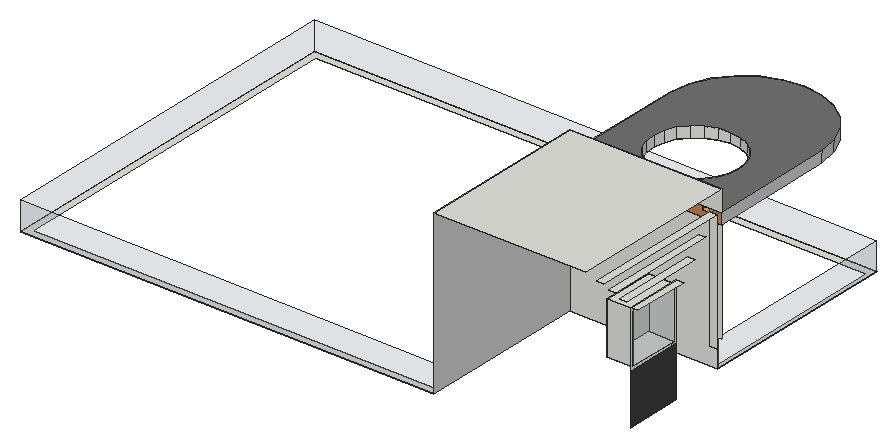
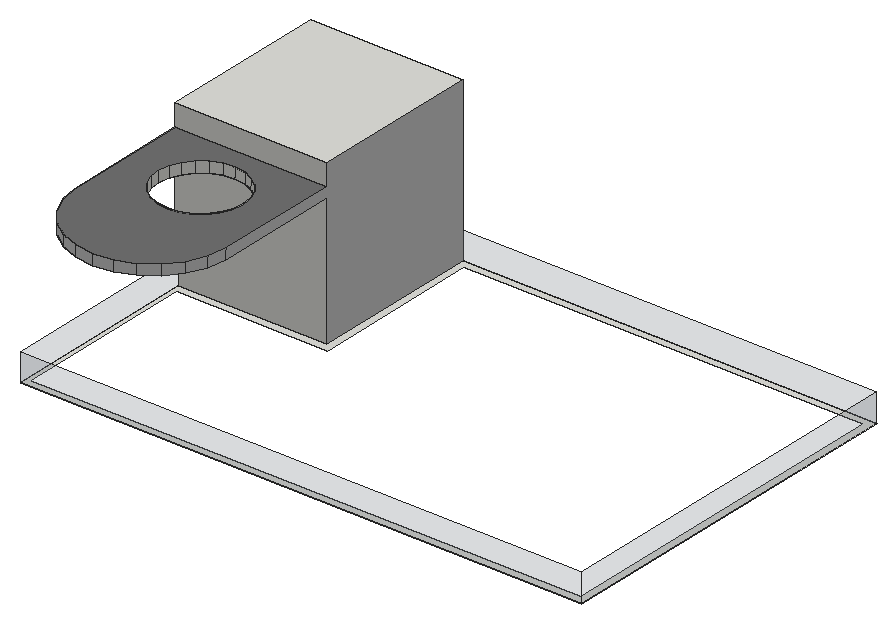
# SketchUp Ruby script. Lengths in inches.
U = 1.inch
M = Sketchup.active_model
def pt(a) = Geom::Point3d.new(a.map { |v| v * U })
def face(e, loops, mat)
  f = e.add_face(loops[0].map { |a| pt(a) })
  loops[1..].each { |l| e.add_face(l.map { |a| pt(a) }).erase! }
  f.material = f.back_material = mat if mat
  f
end
# faces: each face lists its corners as indices into pts; further lists are holes
def faces(e, pts, list, mat = nil) = list.each { |f| face(e, (f[0].is_a?(Array) ? f : [f]).map { |l| l.map { |i| pts[i] } }, mat) }
# xy, xz, yz: faces in a plane at the given z, y or x. An outline is a flat list of corners, or four numbers for a rectangle; further outlines are holes
def ring(l) = l.size == 4 ? [[l[0], l[1]], [l[2], l[1]], [l[2], l[3]], [l[0], l[3]]] : l.each_slice(2).to_a
def flat(e, list, mat, &to3) = list.each { |f| face(e, (f[0].is_a?(Array) ? f : [f]).map { |l| ring(l).map { |u, v| to3.(u, v) } }, mat) }
def xy(e, z, list, mat = nil) = flat(e, list, mat) { |x, y| [x, y, z] }
def xz(e, y, list, mat = nil) = flat(e, list, mat) { |x, z| [x, y, z] }
def yz(e, x, list, mat = nil) = flat(e, list, mat) { |y, z| [x, y, z] }
def lines(e, pts, list) = list.each { |a, b| e.add_line(pt(pts[a]), pt(pts[b])) }
# prism: a flat outline (further loops are holes) pulled along v
def prism(e, loops, v, mat = nil)
  f = face(e, loops, mat); d = Geom::Vector3d.new(v.map { |x| x * U })
  f.pushpull(f.normal.samedirection?(d) ? d.length : -d.length)
end
def box(e, o, s, mat = nil) = prism(e, [[o, [o[0] + s[0], o[1], o[2]], [o[0] + s[0], o[1] + s[1], o[2]], [o[0], o[1] + s[1], o[2]]]], [0, 0, s[2]], mat)
def at(x, y, z, deg = 0) = Geom::Transformation.translation(pt([x, y, z])) * Geom::Transformation.rotation(ORIGIN, Z_AXIS, deg.degrees)
def axes(o, x, y, z) = Geom::Transformation.new([*x, 0, *y, 0, *z, 0, *pt(o).to_a, 1])
def part(name) = M.definitions.add(name)
# library, detail: a bought-in or finely detailed component or shape, given as its bounding box
def library(name, o, s) = part(name).tap { |d| box(d.entities, o, s) }
def detail(e, o, s) = box(e.add_group.entities, o, s)
def put(e, d, t, mat = nil) = e.add_instance(d, t).tap { |i| i.material = mat if mat }
def group(e, t, mat = nil) = e.add_group.tap { |g| g.transformation = t; g.material = mat if mat }.entities
root = M.entities
M.materials.add("Glass_Basic_01").color = [161, 173, 186]
M.materials["Glass_Basic_01"].alpha = 0.25
M.materials.add("M05_Graphite_Haze").color = [114, 114, 114]
M.materials.add("ThomThom - Hat3").color = [58, 58, 58]
M.materials.add("Wood_Veneer_15_1K").color = [173, 116, 75]
M.materials.add("[_0128_White_]").color = [200, 200, 200]
c1 = library("Sphere Light\#1",[-3.43,-3.43,-3.43],[6.86,6.86,6.86])
c2 = library("Sphere Light",[-3.0625,-3.0625,-3.0625],[6.125,6.125,6.125])
c3 = library("Sphere Light\#2",[-2.85,-2.85,-2.85],[5.7,5.7,5.7])
xy(root,270,[[[0,0,351.33,0,351.33,144,477,144,477,312,0,312],[6,6,6,306,474,306,474,150,345.33,150,345.33,6]]])
xy(root,314,[[458.06,50,480,94]])
xy(root,358,[[458.06,50,480,94]])
xy(root,360,[[480,48,486,96]])
xy(root,372,[[480,36,486,108]])
xy(root,381,[[367.15,152.16,367.91,152.34,368.6,152.71,369.17,153.25,369.58,153.92,369.8,154.67,369.82,155.45,369.64,156.21,369.26,156.9,368.73,157.47,368.06,157.88,367.31,158.1,366.52,158.125,365.76,157.94,365.07,157.57,364.51,157.03,364.1,156.36,363.875,155.61,363.85,154.83,364.03,154.07,364.41,153.38,364.95,152.81,365.61,152.4,366.37,152.18],[460.92,152.16,461.68,152.34,462.37,152.71,462.9375,153.25,463.35,153.92,463.57,154.67,463.59,155.45,463.41,156.21,463.03,156.9,462.49,157.47,461.83,157.88,461.08,158.1,460.29,158.125,459.53,157.94,458.84,157.57,458.28,157.03,457.87,156.36,457.64,155.61,457.62,154.83,457.8,154.07,458.18,153.38,458.72,152.81,459.38,152.4,460.13,152.18],[415.67,261.6,416.44,261.71,417.17,262.01,417.79,262.48,418.26,263.1,418.56,263.83,418.67,264.6,418.56,265.38,418.26,266.1,417.79,266.73,417.17,267.2,416.44,267.5,415.67,267.6,414.89,267.5,414.17,267.2,413.55,266.73,413.07,266.1,412.77,265.38,412.67,264.6,412.77,263.83,413.07,263.1,413.55,262.48,414.17,262.01,414.89,261.71]])
xy(root,381,[[[351.33,144,351.33,250.65,354.16,266.71,360.9375,281.55,371.22,294.2,384.35,303.875,399.49,309.94,415.67,312,431.84,309.94,446.98,303.875,460.11,294.2,470.4,281.55,477.17,266.71,480,250.65,480,144],[415.67,161.33,424.98,162.55,433.67,166.15,441.12,171.87,446.84,179.33,450.44,188.01,451.67,197.33,450.44,206.64,446.84,215.33,441.12,222.78,433.67,228.5,424.98,232.1,415.67,233.33,406.35,232.1,397.67,228.5,390.21,222.78,384.49,215.33,380.89,206.64,379.67,197.33,380.89,188.01,384.49,179.33,390.21,171.87,397.67,166.15,406.35,162.55],[409.67,279.92,421.67,291.92]]],"Wood_Veneer_15_1K")
xy(root,384,[[480,24,486,120]])
xy(root,390,[[[351.33,144,480,144,480,250.65,477.17,266.71,470.4,281.55,460.11,294.2,446.98,303.875,431.84,309.94,415.67,312,399.49,309.94,384.35,303.875,371.22,294.2,360.9375,281.55,354.16,266.71,351.33,250.65],[415.67,161.33,406.35,162.55,397.67,166.15,390.21,171.87,384.49,179.33,380.89,188.01,379.67,197.33,380.89,206.64,384.49,215.33,390.21,222.78,397.67,228.5,406.35,232.1,415.67,233.33,424.98,232.1,433.67,228.5,441.12,222.78,446.84,215.33,450.44,206.64,451.67,197.33,450.44,188.01,446.84,179.33,441.12,171.87,433.67,166.15,424.98,162.55]]],"M05_Graphite_Haze")
xy(root,396,[[480,12,486,132]])
xy(root,408,[[351.33,0,480,144]])
xz(root,0,[[0,270,351.33,294]],"Glass_Basic_01")
xz(root,50,[[458.06,314,480,358]])
xz(root,94,[[458.06,314,480,358]])
xz(root,132,[[480,294,486,396]])
xz(root,144,[[351.33,270,351.33,381,480,381,480,294,477,294,477,270],[351.33,390,480,408]])
xz(root,312,[[0,270,477,294]],"Glass_Basic_01")
yz(root,0,[[0,270,312,294]],"Glass_Basic_01")
yz(root,351.33,[[0,270,0,408,144,408,144,390,250.65,390,250.65,381,144,381,144,270]],"[_0128_White_]")
yz(root,458.06,[[50,314,94,358]])
yz(root,477,[[144,270,312,294]],"Glass_Basic_01")
yz(root,480,[[[48,312,96,360],[50,314,94,358]]])
yz(root,480,[[50,314,94,358]],"Glass_Basic_01")
yz(root,480,[[48,268.76,96,312]],"ThomThom - Hat3")
yz(root,480,[[144,381,250.65,390]],"[_0128_White_]")
p = [[406.35,162.55,390],[415.67,161.33,390],[415.67,161.33,381.93],[415.67,161.33,381],[406.35,162.55,381],[424.98,162.55,390],
  [424.98,162.55,381],[397.67,166.15,390],[397.67,166.15,381],[433.67,166.15,390],[433.67,166.15,381],[390.21,171.87,390],
  [390.21,171.87,381],[441.12,171.87,390],[441.12,171.87,381],[384.49,179.33,390],[384.49,179.33,381],[446.84,179.33,390],
  [446.84,179.33,381],[380.89,188.01,390],[380.89,188.01,381],[450.44,188.01,390],[450.44,188.01,381],[379.67,197.33,390],
  [379.67,197.33,381],[451.67,197.33,390],[451.67,197.33,381],[380.89,206.64,390],[380.89,206.64,381],[450.44,206.64,390],
  [450.44,206.64,381],[384.49,215.33,390],[384.49,215.33,381],[446.84,215.33,390],[446.84,215.33,381],[390.21,222.78,390],
  [390.21,222.78,381],[441.12,222.78,390],[441.12,222.78,381],[397.67,228.5,390],[397.67,228.5,381],[433.67,228.5,390],
  [433.67,228.5,381],[406.35,232.1,390],[406.35,232.1,381],[424.98,232.1,390],[424.98,232.1,381],[415.67,233.33,390],
  [415.67,233.33,381],[351.33,250.65,390],[354.16,266.71,390],[354.16,266.71,381],[351.33,250.65,381],[477.17,266.71,390],
  [480,250.65,390],[480,250.65,381],[477.17,266.71,381],[360.9375,281.55,390],[360.9375,281.55,381],[470.4,281.55,390],
  [470.4,281.55,381],[371.22,294.2,390],[371.22,294.2,381],[460.11,294.2,390],[460.11,294.2,381],[384.35,303.875,390],
  [384.35,303.875,381],[446.98,303.875,390],[446.98,303.875,381],[399.49,309.94,390],[399.49,309.94,381],[431.84,309.94,390],
  [431.84,309.94,381],[415.67,312,390],[415.67,312,381],[415.67,144,381]]
faces(root,p,[[0,1,2,3,4],[1,5,6,3,2],[7,0,4,8],[5,9,10,6],[11,7,8,12],[9,13,14,10],[15,11,12,16],[13,17,18,14],
  [19,15,16,20],[17,21,22,18],[23,19,20,24],[21,25,26,22],[27,23,24,28],[25,29,30,26],[31,27,28,32],[29,33,34,30],
  [35,31,32,36],[33,37,38,34],[39,35,36,40],[37,41,42,38],[43,39,40,44],[41,45,46,42],[47,43,44,48],[45,47,48,46]])
faces(root,p,[[49,50,51,52],[53,54,55,56],[50,57,58,51],[59,53,56,60],[57,61,62,58],[63,59,60,64],[61,65,66,62],[67,63,64,68],
  [65,69,70,66],[71,67,68,72],[69,73,74,70],[73,71,72,74]],"[_0128_White_]")
lines(root,p,[[75,2]])
put(root,c1,at(366.55,154.83,381))
put(root,c2,at(460.68,155.01,381))
put(root,c3,at(415.67,264.78,381))
